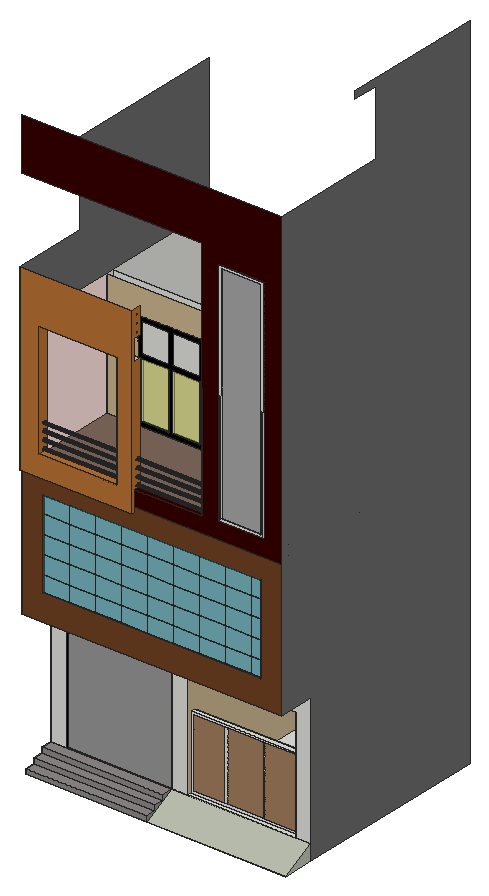
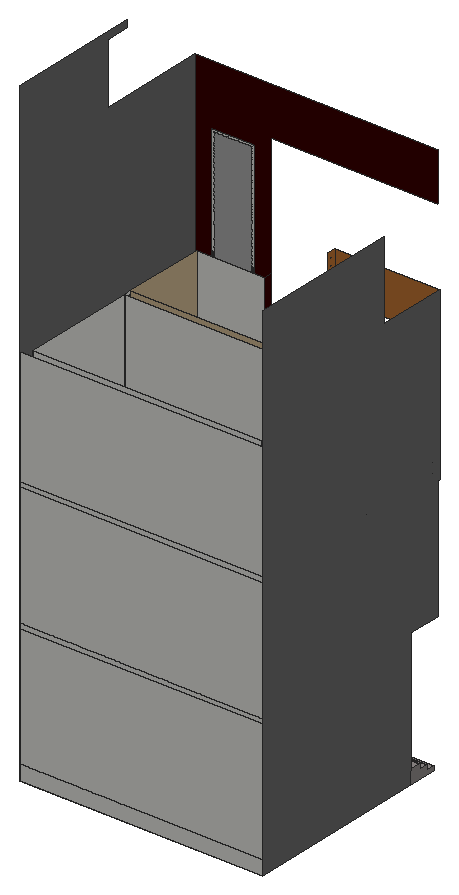
# SketchUp Ruby script. Lengths in inches.
U = 1.inch
M = Sketchup.active_model
def pt(a) = Geom::Point3d.new(a.map { |v| v * U })
def face(e, loops, mat)
  f = e.add_face(loops[0].map { |a| pt(a) })
  loops[1..].each { |l| e.add_face(l.map { |a| pt(a) }).erase! }
  f.material = f.back_material = mat if mat
  f
end
# faces: each face lists its corners as indices into pts; further lists are holes
def faces(e, pts, list, mat = nil) = list.each { |f| face(e, (f[0].is_a?(Array) ? f : [f]).map { |l| l.map { |i| pts[i] } }, mat) }
# xy, xz, yz: faces in a plane at the given z, y or x. An outline is a flat list of corners, or four numbers for a rectangle; further outlines are holes
def ring(l) = l.size == 4 ? [[l[0], l[1]], [l[2], l[1]], [l[2], l[3]], [l[0], l[3]]] : l.each_slice(2).to_a
def flat(e, list, mat, &to3) = list.each { |f| face(e, (f[0].is_a?(Array) ? f : [f]).map { |l| ring(l).map { |u, v| to3.(u, v) } }, mat) }
def xy(e, z, list, mat = nil) = flat(e, list, mat) { |x, y| [x, y, z] }
def xz(e, y, list, mat = nil) = flat(e, list, mat) { |x, z| [x, y, z] }
def yz(e, x, list, mat = nil) = flat(e, list, mat) { |y, z| [x, y, z] }
def lines(e, pts, list) = list.each { |a, b| e.add_line(pt(pts[a]), pt(pts[b])) }
# prism: a flat outline (further loops are holes) pulled along v
def prism(e, loops, v, mat = nil)
  f = face(e, loops, mat); d = Geom::Vector3d.new(v.map { |x| x * U })
  f.pushpull(f.normal.samedirection?(d) ? d.length : -d.length)
end
def box(e, o, s, mat = nil) = prism(e, [[o, [o[0] + s[0], o[1], o[2]], [o[0] + s[0], o[1] + s[1], o[2]], [o[0], o[1] + s[1], o[2]]]], [0, 0, s[2]], mat)
def at(x, y, z, deg = 0) = Geom::Transformation.translation(pt([x, y, z])) * Geom::Transformation.rotation(ORIGIN, Z_AXIS, deg.degrees)
def axes(o, x, y, z) = Geom::Transformation.new([*x, 0, *y, 0, *z, 0, *pt(o).to_a, 1])
def part(name) = M.definitions.add(name)
# library, detail: a bought-in or finely detailed component or shape, given as its bounding box
def library(name, o, s) = part(name).tap { |d| box(d.entities, o, s) }
def detail(e, o, s) = box(e.add_group.entities, o, s)
def put(e, d, t, mat = nil) = e.add_instance(d, t).tap { |i| i.material = mat if mat }
def group(e, t, mat = nil) = e.add_group.tap { |g| g.transformation = t; g.material = mat if mat }.entities
root = M.entities
M.materials.add("[0007_MistyRose]").color = [255, 228, 225]
M.materials.add("[0022_Maroon]").color = [56, 0, 0]
M.materials.add("[0032_Moccasin]").color = [204, 182, 144]
M.materials.add("[0134_DimGray]").color = [105, 105, 105]
M.materials.add("[0137_Black]").color = [0, 0, 0]
M.materials.add("[Checker Plate]").color = [168, 168, 168]
M.materials.add("[Cladding Siding Tan]").color = [162, 126, 95]
M.materials.add("[Cladding Siding White]").color = [153, 153, 153]
M.materials.add("[Granite Brown]").color = [126, 104, 91]
M.materials.add("[Metal Silver]").color = [234, 233, 238]
M.materials.add("[Pavers with Grass Brick]").color = [187, 192, 176]
M.materials.add("[Stone Marble]").color = [143, 138, 136]
M.materials.add("[Translucent Glass Gray]").color = [220, 221, 73]
M.materials["[Translucent Glass Gray]"].alpha = 0.5
M.materials.add("[Translucent Glass Tinted]").color = [5, 136, 163]
M.materials["[Translucent Glass Tinted]"].alpha = 0.48
M.materials.add("[Wood Floor Dark]").color = [186, 114, 51]
M.materials.add("[Wood Veneer 01]").color = [112, 65, 34]
xy(root,-24,[[0,17,278.8125,89],[278.8125,17,600,89],[0,89,600,545]])
xy(root,-12,[[0,17,278.8125,40.0625]],"[Stone Marble]")
xy(root,0,[[0,40.0625,278.8125,62.6875]],"[Stone Marble]")
xy(root,12,[[314.8125,89,564,99.2],[314.8125,99.2,564,109.7],[314.8125,109.7,564,533]])
xy(root,12,[[36,89,278.8125,92]],"[0137_Black]")
xy(root,12,[[0,62.6875,278.8125,89]],"[Stone Marble]")
xy(root,181.25,[[314.8125,99.2,564,109.7]])
xy(root,264,[[36,88,278.8125,92]],"[0137_Black]")
xy(root,271.23,[[314.8125,89,564,533]],"[0032_Moccasin]")
xy(root,285.55,[[36,88,278.8125,89]])
xy(root,312,[[[0,5,600,89],[163.68,35.64,166.79,36.05,169.68,37.25,172.16,39.15,174.07,41.64,175.27,44.53,175.68,47.64,175.27,50.75,174.07,53.64,172.16,56.125,169.68,58.03,166.79,59.23,163.68,59.64,160.57,59.23,157.68,58.03,155.19,56.125,153.29,53.64,152.09,50.75,151.68,47.64,152.09,44.53,153.29,41.64,155.19,39.15,157.68,37.25,160.57,36.05],[55.68,35.64,58.79,36.05,61.68,37.25,64.16,39.15,66.07,41.64,67.27,44.53,67.68,47.64,67.27,50.75,66.07,53.64,64.16,56.125,61.68,58.03,58.79,59.23,55.68,59.64,52.57,59.23,49.68,58.03,47.19,56.125,45.29,53.64,44.09,50.75,43.68,47.64,44.09,44.53,45.29,41.64,47.19,39.15,49.68,37.25,52.57,36.05],[487.68,35.64,490.79,36.05,493.68,37.25,496.16,39.15,498.07,41.64,499.27,44.53,499.68,47.64,499.27,50.75,498.07,53.64,496.16,56.125,493.68,58.03,490.79,59.23,487.68,59.64,484.57,59.23,481.68,58.03,479.19,56.125,477.29,53.64,476.09,50.75,475.68,47.64,476.09,44.53,477.29,41.64,479.19,39.15,481.68,37.25,484.57,36.05],[379.68,35.64,382.79,36.05,385.68,37.25,388.16,39.15,390.07,41.64,391.27,44.53,391.68,47.64,391.27,50.75,390.07,53.64,388.16,56.125,385.68,58.03,382.79,59.23,379.68,59.64,376.57,59.23,373.68,58.03,371.19,56.125,369.29,53.64,368.09,50.75,367.68,47.64,368.09,44.53,369.29,41.64,371.19,39.15,373.68,37.25,376.57,36.05],[271.68,35.64,274.79,36.05,277.68,37.25,280.16,39.15,282.07,41.64,283.27,44.53,283.68,47.64,283.27,50.75,282.07,53.64,280.16,56.125,277.68,58.03,274.79,59.23,271.68,59.64,268.57,59.23,265.68,58.03,263.19,56.125,261.29,53.64,260.09,50.75,259.68,47.64,260.09,44.53,261.29,41.64,263.19,39.15,265.68,37.25,268.57,36.05]],[55.68,35.64,52.57,36.05,49.68,37.25,47.19,39.15,45.29,41.64,44.09,44.53,43.68,47.64,44.09,50.75,45.29,53.64,47.19,56.125,49.68,58.03,52.57,59.23,55.68,59.64,58.79,59.23,61.68,58.03,64.16,56.125,66.07,53.64,67.27,50.75,67.68,47.64,67.27,44.53,66.07,41.64,64.16,39.15,61.68,37.25,58.79,36.05],[163.68,35.64,160.57,36.05,157.68,37.25,155.19,39.15,153.29,41.64,152.09,44.53,151.68,47.64,152.09,50.75,153.29,53.64,155.19,56.125,157.68,58.03,160.57,59.23,163.68,59.64,166.79,59.23,169.68,58.03,172.16,56.125,174.07,53.64,175.27,50.75,175.68,47.64,175.27,44.53,174.07,41.64,172.16,39.15,169.68,37.25,166.79,36.05],[271.68,35.64,268.57,36.05,265.68,37.25,263.19,39.15,261.29,41.64,260.09,44.53,259.68,47.64,260.09,50.75,261.29,53.64,263.19,56.125,265.68,58.03,268.57,59.23,271.68,59.64,274.79,59.23,277.68,58.03,280.16,56.125,282.07,53.64,283.27,50.75,283.68,47.64,283.27,44.53,282.07,41.64,280.16,39.15,277.68,37.25,274.79,36.05],[379.68,35.64,376.57,36.05,373.68,37.25,371.19,39.15,369.29,41.64,368.09,44.53,367.68,47.64,368.09,50.75,369.29,53.64,371.19,56.125,373.68,58.03,376.57,59.23,379.68,59.64,382.79,59.23,385.68,58.03,388.16,56.125,390.07,53.64,391.27,50.75,391.68,47.64,391.27,44.53,390.07,41.64,388.16,39.15,385.68,37.25,382.79,36.05],
  [487.68,35.64,484.57,36.05,481.68,37.25,479.19,39.15,477.29,41.64,476.09,44.53,475.68,47.64,476.09,50.75,477.29,53.64,479.19,56.125,481.68,58.03,484.57,59.23,487.68,59.64,490.79,59.23,493.68,58.03,496.16,56.125,498.07,53.64,499.27,50.75,499.68,47.64,499.27,44.53,498.07,41.64,496.16,39.15,493.68,37.25,490.79,36.05]])
xy(root,324,[[18,23,582,527]])
xy(root,372,[[48,5,552,8]],"[Wood Veneer 01]")
xy(root,576,[[48,5,552,8]],"[Wood Veneer 01]")
xy(root,612,[[0,0,258,5]],"[Wood Floor Dark]")
xy(root,636,[[18,227,582,245],[18,245,582,527]])
xy(root,636,[[18,23,582,227]],"[Granite Brown]")
xy(root,645.8125,[[98.58,227,160.58,229],[170.58,227,232.58,229],[242.58,227,307.71,229]])
xy(root,660,[[258,5,414,23]],"[0022_Maroon]")
xy(root,660,[[42,0,222,23]],"[Wood Floor Dark]")
xy(root,665.86,[[455.86,3,558.14,5]])
xy(root,670.74,[[460.74,3,553.26,5]])
xy(root,704.4,[[370.68,227,426.27,229],[434.59,227,482.8,229]])
xz(root,0,[[[0,612,258,1032],[42,660,222,924]]],"[Wood Floor Dark]")
xz(root,3,[[[455.86,665.86,558.14,1194.14],[460.74,670.74,553.26,1189.26]]])
xz(root,5,[[[455.86,665.86,558.14,1194.14],[460.74,670.74,553.26,1189.26]]])
xz(root,5,[[[258,624,600,624,600,1344,0,1344,0,1224,414,1224,414,660,258,660],[455.86,665.86,558.14,1194.14]]],"[0022_Maroon]")
xz(root,5,[[460.74,670.74,553.26,1189.26]],"[Checker Plate]")
xz(root,5,[[[0,312,600,312,600,624,258,624,258,612,0,612],[48,372,552,576]]],"[Wood Veneer 01]")
xz(root,8,[[48,372,108,408],[108,372,168,408],[168,372,228,408],[228,372,288,408],[288,372,348,408],
  [348,372,408,408],[408,372,468,408],[468,372,528,408],[528,372,552,408],[48,408,108,450],
  [108,408,168,450],[168,408,228,450],[228,408,288,450],[288,408,348,450],[348,408,408,450],
  [408,408,468,450],[468,408,528,450],[528,408,552,450],[48,450,108,492],[108,450,168,492],
  [168,450,228,492],[228,450,288,492],[288,450,348,492],[348,450,408,492],[408,450,468,492],
  [468,450,528,492],[528,450,552,492],[48,492,108,534],[108,492,168,534],[168,492,228,534],
  [228,492,288,534],[288,492,348,534],[348,492,408,534],[408,492,468,534],[468,492,528,534],
  [528,492,552,534],[48,534,108,576],[108,534,168,576],[168,534,228,576],[228,534,288,576],
  [288,534,348,576],[348,534,408,576],[408,534,468,576],[468,534,528,576],[528,534,552,576]],"[Translucent Glass Tinted]")
xz(root,17,[[0,-24,278.8125,-12]],"[Stone Marble]")
xz(root,23,[[18,324,582,624],[18,636,582,660],[18,660,42,924],[222,660,258,924],[414,660,582,924]])
xz(root,40.0625,[[0,-12,278.8125,0]],"[Stone Marble]")
xz(root,62.6875,[[0,0,278.8125,12]],"[Stone Marble]")
xz(root,88,[[36,264,278.8125,285.55]],"[0137_Black]")
xz(root,89,[[0,-24,278.8125,-12],[278.8125,-24,600,12],[0,-12,278.8125,0],[0,0,278.8125,12],[0,12,36,12,36,285.55,278.8125,285.55,278.8125,12,314.8125,12,314.8125,271.23,564,271.23,564,12,600,12,600,312,0,312]])
xz(root,92,[[36,12,278.8125,264]],"[Cladding Siding White]")
xz(root,99.2,[[392.8125,18,398.8125,175.25]])
xz(root,99.2,[[320.8125,18,392.8125,175.25],[398.8125,18,479.75,175.25],[485.75,18,558,175.25]],"[Cladding Siding Tan]")
xz(root,99.2,[[[314.8125,12,564,181.25],[320.8125,18,558,175.25]],[479.75,18,485.75,175.25]],"[Metal Silver]")
xz(root,109.7,[[314.8125,12,564,181.25]])
xz(root,227,[[[18,636,88.77,636,88.77,864.75,317.52,864.75,317.52,636,582,636,582,924,18,924],[361.58,695.31,491.89,865.62]]],"[0032_Moccasin]")
xz(root,227,[[[88.77,636,317.52,864.75],[242.58,645.8125,307.71,776.75],[98.58,645.8125,160.58,776.75],[170.58,645.8125,232.58,776.75],[242.58,786.75,307.71,854.9375],[170.58,786.75,232.58,854.9375],[98.58,786.75,160.58,854.9375]],[[361.58,695.31,491.89,865.62],[370.68,704.4,482.8,856.52]],[426.27,704.4,434.59,856.52]],"[0137_Black]")
xz(root,229,[[98.58,645.8125,160.58,776.75],[170.58,645.8125,232.58,776.75],[242.58,645.8125,307.71,776.75],[370.68,704.4,426.27,856.52],[434.59,704.4,482.8,856.52]],"[Translucent Glass Gray]")
xz(root,245,[[18,636,582,924]])
xz(root,527,[[18,324,582,624],[18,636,582,924]])
xz(root,533,[[314.8125,12,564,271.23]],"[0032_Moccasin]")
xz(root,545,[[0,-24,600,12],[0,12,600,312],[0,312,600,324],[0,324,600,624],[0,624,600,636],
  [0,636,600,924]])
yz(root,0,[[89,-24,89,312,5,312,5,612,0,612,0,1032,173,1032,173,1224,545,1224,545,-24]],"[0134_DimGray]")
yz(root,0,[[17,-24,17,-12,40.0625,-12,40.0625,0,62.6875,0,62.6875,12,89,12,89,-24]],"[Stone Marble]")
yz(root,18,[[23,324,527,624],[227,636,245,924],[245,636,527,924]])
yz(root,18,[[23,636,227,924]],"[0007_MistyRose]")
yz(root,36,[[88,264,89,285.55]])
yz(root,36,[[89,12,92,264]],"[0137_Black]")
yz(root,42,[[14,663,13.22,663.1,12.5,663.4,11.88,663.88,11.4,664.5,11.1,665.22,11,666,11.1,666.78,11.4,667.5,11.88,668.12,12.5,668.6,13.22,668.9,14,669,14.78,668.9,15.5,668.6,16.12,668.12,16.6,667.5,16.9,666.78,17,666,16.9,665.22,16.6,664.5,16.12,663.88,15.5,663.4,14.78,663.1],[14,681,13.22,681.1,12.5,681.4,11.88,681.88,11.4,682.5,11.1,683.22,11,684,11.1,684.78,11.4,685.5,11.88,686.12,12.5,686.6,13.22,686.9,14,687,14.78,686.9,15.5,686.6,16.12,686.12,16.6,685.5,16.9,684.78,17,684,16.9,683.22,16.6,682.5,16.12,681.88,15.5,681.4,14.78,681.1],[14,699,13.22,699.1,12.5,699.4,11.88,699.88,11.4,700.5,11.1,701.22,11,702,11.1,702.78,11.4,703.5,11.88,704.12,12.5,704.6,13.22,704.9,14,705,14.78,704.9,15.5,704.6,16.12,704.12,16.6,703.5,16.9,702.78,17,702,16.9,701.22,16.6,700.5,16.12,699.88,15.5,699.4,14.78,699.1],[14,717,13.22,717.1,12.5,717.4,11.88,717.88,11.4,718.5,11.1,719.22,11,720,11.1,720.78,11.4,721.5,11.88,722.12,12.5,722.6,13.22,722.9,14,723,14.78,722.9,15.5,722.6,16.12,722.12,16.6,721.5,16.9,720.78,17,720,16.9,719.22,16.6,718.5,16.12,717.88,15.5,717.4,14.78,717.1]])
yz(root,42,[[[0,660,23,924],[14,717,13.22,717.1,12.5,717.4,11.88,717.88,11.4,718.5,11.1,719.22,11,720,11.1,720.78,11.4,721.5,11.88,722.12,12.5,722.6,13.22,722.9,14,723,14.78,722.9,15.5,722.6,16.12,722.12,16.6,721.5,16.9,720.78,17,720,16.9,719.22,16.6,718.5,16.12,717.88,15.5,717.4,14.78,717.1],[14,699,13.22,699.1,12.5,699.4,11.88,699.88,11.4,700.5,11.1,701.22,11,702,11.1,702.78,11.4,703.5,11.88,704.12,12.5,704.6,13.22,704.9,14,705,14.78,704.9,15.5,704.6,16.12,704.12,16.6,703.5,16.9,702.78,17,702,16.9,701.22,16.6,700.5,16.12,699.88,15.5,699.4,14.78,699.1],[14,681,13.22,681.1,12.5,681.4,11.88,681.88,11.4,682.5,11.1,683.22,11,684,11.1,684.78,11.4,685.5,11.88,686.12,12.5,686.6,13.22,686.9,14,687,14.78,686.9,15.5,686.6,16.12,686.12,16.6,685.5,16.9,684.78,17,684,16.9,683.22,16.6,682.5,16.12,681.88,15.5,681.4,14.78,681.1],[14,663,13.22,663.1,12.5,663.4,11.88,663.88,11.4,664.5,11.1,665.22,11,666,11.1,666.78,11.4,667.5,11.88,668.12,12.5,668.6,13.22,668.9,14,669,14.78,668.9,15.5,668.6,16.12,668.12,16.6,667.5,16.9,666.78,17,666,16.9,665.22,16.6,664.5,16.12,663.88,15.5,663.4,14.78,663.1]]],"[Wood Floor Dark]")
yz(root,48,[[5,372,8,576]],"[Wood Veneer 01]")
yz(root,98.58,[[227,645.8125,229,776.75]])
yz(root,160.58,[[227,645.8125,229,776.75]])
yz(root,170.58,[[227,645.8125,229,776.75]])
yz(root,222,[[[0,660,23,924],[14,717,14.78,717.1,15.5,717.4,16.12,717.88,16.6,718.5,16.9,719.22,17,720,16.9,720.78,16.6,721.5,16.12,722.12,15.5,722.6,14.78,722.9,14,723,13.22,722.9,12.5,722.6,11.88,722.12,11.4,721.5,11.1,720.78,11,720,11.1,719.22,11.4,718.5,11.88,717.88,12.5,717.4,13.22,717.1],[14,699,14.78,699.1,15.5,699.4,16.12,699.88,16.6,700.5,16.9,701.22,17,702,16.9,702.78,16.6,703.5,16.12,704.12,15.5,704.6,14.78,704.9,14,705,13.22,704.9,12.5,704.6,11.88,704.12,11.4,703.5,11.1,702.78,11,702,11.1,701.22,11.4,700.5,11.88,699.88,12.5,699.4,13.22,699.1],[14,681,14.78,681.1,15.5,681.4,16.12,681.88,16.6,682.5,16.9,683.22,17,684,16.9,684.78,16.6,685.5,16.12,686.12,15.5,686.6,14.78,686.9,14,687,13.22,686.9,12.5,686.6,11.88,686.12,11.4,685.5,11.1,684.78,11,684,11.1,683.22,11.4,682.5,11.88,681.88,12.5,681.4,13.22,681.1],[14,663,14.78,663.1,15.5,663.4,16.12,663.88,16.6,664.5,16.9,665.22,17,666,16.9,666.78,16.6,667.5,16.12,668.12,15.5,668.6,14.78,668.9,14,669,13.22,668.9,12.5,668.6,11.88,668.12,11.4,667.5,11.1,666.78,11,666,11.1,665.22,11.4,664.5,11.88,663.88,12.5,663.4,13.22,663.1]]],"[Wood Floor Dark]")
yz(root,232.58,[[227,645.8125,229,776.75]])
yz(root,242.58,[[227,645.8125,229,776.75]])
yz(root,258,[[14,663,13.22,663.1,12.5,663.4,11.88,663.88,11.4,664.5,11.1,665.22,11,666,11.1,666.78,11.4,667.5,11.88,668.12,12.5,668.6,13.22,668.9,14,669,14.78,668.9,15.5,668.6,16.12,668.12,16.6,667.5,16.9,666.78,17,666,16.9,665.22,16.6,664.5,16.12,663.88,15.5,663.4,14.78,663.1],[14,681,13.22,681.1,12.5,681.4,11.88,681.88,11.4,682.5,11.1,683.22,11,684,11.1,684.78,11.4,685.5,11.88,686.12,12.5,686.6,13.22,686.9,14,687,14.78,686.9,15.5,686.6,16.12,686.12,16.6,685.5,16.9,684.78,17,684,16.9,683.22,16.6,682.5,16.12,681.88,15.5,681.4,14.78,681.1],[14,699,13.22,699.1,12.5,699.4,11.88,699.88,11.4,700.5,11.1,701.22,11,702,11.1,702.78,11.4,703.5,11.88,704.12,12.5,704.6,13.22,704.9,14,705,14.78,704.9,15.5,704.6,16.12,704.12,16.6,703.5,16.9,702.78,17,702,16.9,701.22,16.6,700.5,16.12,699.88,15.5,699.4,14.78,699.1],[14,717,13.22,717.1,12.5,717.4,11.88,717.88,11.4,718.5,11.1,719.22,11,720,11.1,720.78,11.4,721.5,11.88,722.12,12.5,722.6,13.22,722.9,14,723,14.78,722.9,15.5,722.6,16.12,722.12,16.6,721.5,16.9,720.78,17,720,16.9,719.22,16.6,718.5,16.12,717.88,15.5,717.4,14.78,717.1]])
yz(root,258,[[[0,612,5,612,5,660,23,660,23,924,5,924,5,972,23,972,23,1032,0,1032],[14,977.83,13.63,977.85,13.27,977.91,12.92,978,12.57,978.14,12.25,978.3,11.9375,978.5,11.65,978.73,11.39,978.99,11.16,979.28,10.96,979.59,10.8,979.91,10.66,980.26,10.57,980.61,10.51,980.97,10.49,981.34,10.51,981.71,10.57,982.07,10.66,982.42,10.8,982.77,10.96,983.09,11.16,983.4,11.39,983.6875,11.65,983.95,11.9375,984.18,12.25,984.38,12.57,984.54,12.92,984.68,13.27,984.77,13.63,984.83,14,984.85,14.37,984.83,14.73,984.77,15.08,984.68,15.43,984.54,15.75,984.38,16.0625,984.18,16.35,983.95,16.61,983.6875,16.84,983.4,17.04,983.09,17.2,982.77,17.34,982.42,17.43,982.07,17.49,981.71,17.51,981.34,17.49,980.97,17.43,980.61,17.34,980.26,17.2,979.91,17.04,979.59,16.84,979.28,16.61,978.99,16.35,978.73,16.0625,978.5,15.75,978.3,15.43,978.14,15.08,978,14.73,977.91,14.37,977.85],[14,1013.83,13.63,1013.85,13.27,1013.91,12.92,1014.01,12.57,1014.14,12.25,1014.3,11.9375,1014.5,11.65,1014.74,11.39,1014.99,11.16,1015.28,10.96,1015.59,10.8,1015.91,10.67,1016.26,10.57,1016.61,10.51,1016.97,10.49,1017.34,10.51,1017.71,10.57,1018.07,10.67,1018.42,10.8,1018.77,10.96,1019.09,11.16,1019.4,11.39,1019.6875,11.65,1019.95,11.9375,1020.18,12.25,1020.375,12.57,1020.54,12.92,1020.68,13.27,1020.77,13.63,1020.83,14,1020.85,14.37,1020.83,14.73,1020.77,15.08,1020.68,15.43,1020.54,15.75,1020.375,16.0625,1020.18,16.35,1019.95,16.61,1019.6875,16.84,1019.4,17.04,1019.09,17.2,1018.77,17.33,1018.42,17.43,1018.07,17.49,1017.71,17.51,1017.34,17.49,1016.97,17.43,1016.61,17.33,1016.26,17.2,1015.91,17.04,1015.59,16.84,1015.28,16.61,1014.99,16.35,1014.74,16.0625,1014.5,15.75,1014.3,15.43,1014.14,15.08,1014.01,14.73,1013.91,14.37,1013.85],[14,996.07,13.66,996.09,13.32,996.14,12.99,996.23,12.67,996.35,12.36,996.51,12.08,996.69,11.81,996.91,11.57,997.15,11.35,997.42,11.17,997.7,11.01,998.01,10.89,998.33,10.8,998.66,10.75,999,10.73,999.34,10.75,999.68,10.8,1000.02,10.89,1000.35,11.01,1000.67,11.17,1000.98,11.35,1001.26,11.57,1001.53,11.81,1001.77,12.08,1001.99,12.36,1002.17,12.67,1002.33,12.99,1002.45,13.32,1002.54,13.66,1002.6,14,1002.61,14.34,1002.6,14.68,1002.54,15.01,1002.45,15.33,1002.33,15.64,1002.17,15.92,1001.99,16.19,1001.77,16.43,1001.53,16.65,1001.26,16.83,1000.98,16.99,1000.67,17.11,1000.35,17.2,1000.02,17.25,999.68,17.27,999.34,17.25,999,17.2,998.66,17.11,998.33,16.99,998.01,16.83,997.7,16.65,997.42,16.43,997.15,16.19,996.91,15.92,996.69,15.64,996.51,15.33,996.35,15.01,996.23,14.68,996.14,14.34,996.09],[14,717,13.22,717.1,12.5,717.4,11.88,717.88,11.4,718.5,11.1,719.22,11,720,11.1,720.78,11.4,721.5,11.88,722.12,12.5,722.6,13.22,722.9,14,723,14.78,722.9,15.5,722.6,16.12,722.12,16.6,721.5,16.9,720.78,17,720,16.9,719.22,16.6,718.5,16.12,717.88,15.5,717.4,14.78,717.1],[14,699,13.22,699.1,12.5,699.4,11.88,699.88,11.4,700.5,11.1,701.22,11,702,11.1,702.78,11.4,703.5,11.88,704.12,12.5,704.6,13.22,704.9,14,705,14.78,704.9,15.5,704.6,16.12,704.12,16.6,703.5,16.9,702.78,17,702,16.9,701.22,16.6,700.5,16.12,699.88,15.5,699.4,14.78,699.1],[14,681,13.22,681.1,12.5,681.4,11.88,681.88,11.4,682.5,11.1,683.22,11,684,11.1,684.78,11.4,685.5,11.88,686.12,12.5,686.6,13.22,686.9,14,687,14.78,686.9,15.5,686.6,16.12,686.12,16.6,685.5,16.9,684.78,17,684,16.9,683.22,16.6,682.5,16.12,681.88,15.5,681.4,14.78,681.1],[14,663,13.22,663.1,12.5,663.4,11.88,663.88,11.4,664.5,11.1,665.22,11,666,11.1,666.78,11.4,667.5,11.88,668.12,12.5,668.6,13.22,668.9,14,669,14.78,668.9,15.5,668.6,16.12,668.12,16.6,667.5,16.9,666.78,17,666,16.9,665.22,16.6,664.5,16.12,663.88,15.5,663.4,14.78,663.1]]],"[Wood Floor Dark]")
yz(root,278.8125,[[88,264,89,285.55]])
yz(root,278.8125,[[89,12,92,264]],"[0137_Black]")
yz(root,278.8125,[[17,-24,89,12,62.6875,12,62.6875,0,40.0625,0,40.0625,-12,17,-12]],"[Stone Marble]")
yz(root,307.71,[[227,645.8125,229,776.75]])
yz(root,314.8125,[[89,12,99.2,12,99.2,181.25,109.7,181.25,109.7,12,533,12,533,271.23,89,271.23]],"[0032_Moccasin]")
yz(root,370.68,[[227,704.4,229,856.52]])
yz(root,414,[[[5,660,23,924],[14,717,14.78,717.1,15.5,717.4,16.12,717.88,16.6,718.5,16.9,719.22,17,720,16.9,720.78,16.6,721.5,16.12,722.12,15.5,722.6,14.78,722.9,14,723,13.22,722.9,12.5,722.6,11.88,722.12,11.4,721.5,11.1,720.78,11,720,11.1,719.22,11.4,718.5,11.88,717.88,12.5,717.4,13.22,717.1],[14,699,14.78,699.1,15.5,699.4,16.12,699.88,16.6,700.5,16.9,701.22,17,702,16.9,702.78,16.6,703.5,16.12,704.12,15.5,704.6,14.78,704.9,14,705,13.22,704.9,12.5,704.6,11.88,704.12,11.4,703.5,11.1,702.78,11,702,11.1,701.22,11.4,700.5,11.88,699.88,12.5,699.4,13.22,699.1],[14,681,14.78,681.1,15.5,681.4,16.12,681.88,16.6,682.5,16.9,683.22,17,684,16.9,684.78,16.6,685.5,16.12,686.12,15.5,686.6,14.78,686.9,14,687,13.22,686.9,12.5,686.6,11.88,686.12,11.4,685.5,11.1,684.78,11,684,11.1,683.22,11.4,682.5,11.88,681.88,12.5,681.4,13.22,681.1],[14,663,14.78,663.1,15.5,663.4,16.12,663.88,16.6,664.5,16.9,665.22,17,666,16.9,666.78,16.6,667.5,16.12,668.12,15.5,668.6,14.78,668.9,14,669,13.22,668.9,12.5,668.6,11.88,668.12,11.4,667.5,11.1,666.78,11,666,11.1,665.22,11.4,664.5,11.88,663.88,12.5,663.4,13.22,663.1]]],"[0022_Maroon]")
yz(root,426.27,[[227,704.4,229,856.52]])
yz(root,434.59,[[227,704.4,229,856.52]])
yz(root,455.86,[[3,665.86,5,924]])
yz(root,460.74,[[3,670.74,5,924]])
yz(root,482.8,[[227,704.4,229,856.52]])
yz(root,552,[[5,372,8,576]],"[Wood Veneer 01]")
yz(root,553.26,[[3,670.74,5,924]])
yz(root,558.14,[[3,665.86,5,924]])
yz(root,564,[[99.2,12,109.7,181.25]])
yz(root,564,[[89,12,89,271.23,533,271.23,533,12,109.7,12,109.7,181.25,99.2,181.25,99.2,12]],"[0032_Moccasin]")
yz(root,582,[[23,324,527,624],[227,636,245,924],[245,636,527,924]])
yz(root,582,[[23,636,227,924]],"[0032_Moccasin]")
yz(root,600,[[89,-24,545,-24,545,1512,215,1512,215,1494,275,1494,275,1344,5,1344,5,312,89,312]],"[0134_DimGray]")
yz(root,600,[[17,-24,89,-24,89,12]],"[Pavers with Grass Brick]")
p = [[600,17,-24],[600,89,12],[564,89,12],[314.8125,89,12],[278.8125,89,12],[278.8125,17,-24],
  [42,13.22,663.1],[42,14,663],[222,14,663],[222,13.22,663.1],[258,13.22,663.1],[258,14,663],
  [414,14,663],[414,13.22,663.1],[42,14.78,663.1],[222,14.78,663.1],[258,14.78,663.1],[414,14.78,663.1],
  [42,12.5,663.4],[222,12.5,663.4],[258,12.5,663.4],[414,12.5,663.4],[42,15.5,663.4],[222,15.5,663.4],
  [258,15.5,663.4],[414,15.5,663.4],[42,11.88,663.88],[222,11.88,663.88],[258,11.88,663.88],[414,11.88,663.88],
  [42,16.12,663.88],[222,16.12,663.88],[258,16.12,663.88],[414,16.12,663.88],[42,11.4,664.5],[222,11.4,664.5],
  [258,11.4,664.5],[414,11.4,664.5],[42,16.6,664.5],[222,16.6,664.5],[258,16.6,664.5],[414,16.6,664.5],
  [42,11.1,665.22],[222,11.1,665.22],[258,11.1,665.22],[414,11.1,665.22],[42,16.9,665.22],[222,16.9,665.22],
  [258,16.9,665.22],[414,16.9,665.22],[42,11,666],[222,11,666],[258,11,666],[414,11,666],
  [42,17,666],[222,17,666],[258,17,666],[414,17,666],[42,11.1,666.78],[222,11.1,666.78],
  [258,11.1,666.78],[414,11.1,666.78],[42,16.9,666.78],[222,16.9,666.78],[258,16.9,666.78],[414,16.9,666.78],
  [42,11.4,667.5],[222,11.4,667.5],[258,11.4,667.5],[414,11.4,667.5],[42,16.6,667.5],[222,16.6,667.5],
  [258,16.6,667.5],[414,16.6,667.5],[42,11.88,668.12],[222,11.88,668.12],[258,11.88,668.12],[414,11.88,668.12],
  [42,16.12,668.12],[222,16.12,668.12],[258,16.12,668.12],[414,16.12,668.12],[42,12.5,668.6],[222,12.5,668.6],
  [258,12.5,668.6],[414,12.5,668.6],[42,15.5,668.6],[222,15.5,668.6],[258,15.5,668.6],[414,15.5,668.6],
  [42,13.22,668.9],[222,13.22,668.9],[258,13.22,668.9],[414,13.22,668.9],[42,14.78,668.9],[222,14.78,668.9],
  [258,14.78,668.9],[414,14.78,668.9],[42,14,669],[222,14,669],[258,14,669],[414,14,669],
  [42,13.22,681.1],[42,14,681],[222,14,681],[222,13.22,681.1],[258,13.22,681.1],[258,14,681],
  [414,14,681],[414,13.22,681.1],[42,14.78,681.1],[222,14.78,681.1],[258,14.78,681.1],[414,14.78,681.1],
  [42,12.5,681.4],[222,12.5,681.4],[258,12.5,681.4],[414,12.5,681.4],[42,15.5,681.4],[222,15.5,681.4],
  [258,15.5,681.4],[414,15.5,681.4],[42,11.88,681.88],[222,11.88,681.88],[258,11.88,681.88],[414,11.88,681.88],
  [42,16.12,681.88],[222,16.12,681.88],[258,16.12,681.88],[414,16.12,681.88],[42,11.4,682.5],[222,11.4,682.5],
  [258,11.4,682.5],[414,11.4,682.5],[42,16.6,682.5],[222,16.6,682.5],[258,16.6,682.5],[414,16.6,682.5],
  [42,11.1,683.22],[222,11.1,683.22],[258,11.1,683.22],[414,11.1,683.22],[42,16.9,683.22],[222,16.9,683.22],
  [258,16.9,683.22],[414,16.9,683.22],[42,11,684],[222,11,684],[258,11,684],[414,11,684],
  [42,17,684],[222,17,684],[258,17,684],[414,17,684],[42,11.1,684.78],[222,11.1,684.78],
  [258,11.1,684.78],[414,11.1,684.78],[42,16.9,684.78],[222,16.9,684.78],[258,16.9,684.78],[414,16.9,684.78],
  [42,11.4,685.5],[222,11.4,685.5],[258,11.4,685.5],[414,11.4,685.5],[42,16.6,685.5],[222,16.6,685.5],
  [258,16.6,685.5],[414,16.6,685.5],[42,11.88,686.12],[222,11.88,686.12],[258,11.88,686.12],[414,11.88,686.12],
  [42,16.12,686.12],[222,16.12,686.12],[258,16.12,686.12],[414,16.12,686.12],[42,12.5,686.6],[222,12.5,686.6],
  [258,12.5,686.6],[414,12.5,686.6],[42,15.5,686.6],[222,15.5,686.6],[258,15.5,686.6],[414,15.5,686.6],
  [42,13.22,686.9],[222,13.22,686.9],[258,13.22,686.9],[414,13.22,686.9],[42,14.78,686.9],[222,14.78,686.9],
  [258,14.78,686.9],[414,14.78,686.9],[42,14,687],[222,14,687],[258,14,687],[414,14,687],
  [42,13.22,699.1],[42,14,699],[222,14,699],[222,13.22,699.1],[258,13.22,699.1],[258,14,699],
  [414,14,699],[414,13.22,699.1],[42,14.78,699.1],[222,14.78,699.1],[258,14.78,699.1],[414,14.78,699.1],
  [42,12.5,699.4],[222,12.5,699.4],[258,12.5,699.4],[414,12.5,699.4],[42,15.5,699.4],[222,15.5,699.4],
  [258,15.5,699.4],[414,15.5,699.4],[42,11.88,699.88],[222,11.88,699.88],[258,11.88,699.88],[414,11.88,699.88],
  [42,16.12,699.88],[222,16.12,699.88],[258,16.12,699.88],[414,16.12,699.88],[42,11.4,700.5],[222,11.4,700.5],
  [258,11.4,700.5],[414,11.4,700.5],[42,16.6,700.5],[222,16.6,700.5],[258,16.6,700.5],[414,16.6,700.5],
  [42,11.1,701.22],[222,11.1,701.22],[258,11.1,701.22],[414,11.1,701.22],[42,16.9,701.22],[222,16.9,701.22],
  [258,16.9,701.22],[414,16.9,701.22],[42,11,702],[222,11,702],[258,11,702],[414,11,702],
  [42,17,702],[222,17,702],[258,17,702],[414,17,702],[42,11.1,702.78],[222,11.1,702.78],
  [258,11.1,702.78],[414,11.1,702.78],[42,16.9,702.78],[222,16.9,702.78],[258,16.9,702.78],[414,16.9,702.78],
  [42,11.4,703.5],[222,11.4,703.5],[258,11.4,703.5],[414,11.4,703.5],[42,16.6,703.5],[222,16.6,703.5],
  [258,16.6,703.5],[414,16.6,703.5],[42,11.88,704.12],[222,11.88,704.12],[258,11.88,704.12],[414,11.88,704.12],
  [42,16.12,704.12],[222,16.12,704.12],[258,16.12,704.12],[414,16.12,704.12],[42,12.5,704.6],[222,12.5,704.6],
  [258,12.5,704.6],[414,12.5,704.6],[42,15.5,704.6],[222,15.5,704.6],[258,15.5,704.6],[414,15.5,704.6],
  [42,13.22,704.9],[222,13.22,704.9],[258,13.22,704.9],[414,13.22,704.9],[42,14.78,704.9],[222,14.78,704.9],
  [258,14.78,704.9],[414,14.78,704.9],[42,14,705],[222,14,705],[258,14,705],[414,14,705],
  [42,13.22,717.1],[42,14,717],[222,14,717],[222,13.22,717.1],[258,13.22,717.1],[258,14,717],
  [414,14,717],[414,13.22,717.1],[42,14.78,717.1],[222,14.78,717.1],[258,14.78,717.1],[414,14.78,717.1],
  [42,12.5,717.4],[222,12.5,717.4],[258,12.5,717.4],[414,12.5,717.4],[42,15.5,717.4],[222,15.5,717.4],
  [258,15.5,717.4],[414,15.5,717.4],[42,11.88,717.88],[222,11.88,717.88],[258,11.88,717.88],[414,11.88,717.88],
  [42,16.12,717.88],[222,16.12,717.88],[258,16.12,717.88],[414,16.12,717.88],[42,11.4,718.5],[222,11.4,718.5],
  [258,11.4,718.5],[414,11.4,718.5],[42,16.6,718.5],[222,16.6,718.5],[258,16.6,718.5],[414,16.6,718.5],
  [42,11.1,719.22],[222,11.1,719.22],[258,11.1,719.22],[414,11.1,719.22],[42,16.9,719.22],[222,16.9,719.22],
  [258,16.9,719.22],[414,16.9,719.22],[42,11,720],[222,11,720],[258,11,720],[414,11,720],
  [42,17,720],[222,17,720],[258,17,720],[414,17,720],[42,11.1,720.78],[222,11.1,720.78],
  [258,11.1,720.78],[414,11.1,720.78],[42,16.9,720.78],[222,16.9,720.78],[258,16.9,720.78],[414,16.9,720.78],
  [42,11.4,721.5],[222,11.4,721.5],[258,11.4,721.5],[414,11.4,721.5],[42,16.6,721.5],[222,16.6,721.5],
  [258,16.6,721.5],[414,16.6,721.5],[42,11.88,722.12],[222,11.88,722.12],[258,11.88,722.12],[414,11.88,722.12],
  [42,16.12,722.12],[222,16.12,722.12],[258,16.12,722.12],[414,16.12,722.12],[18,23,636],[0,23,636],
  [582,23,636],[600,23,636],[0,227,636],[18,227,636],[582,227,636],[600,227,636],
  [582,23,660],[600,23,660],[18,23,660],[0,23,660],[588,8,372],[588,8,576],
  [258,14,666],[414,14,666],[258,14,684],[414,14,684],[258,14,702],[414,14,702],
  [258,14,720],[414,14,720],[42,14,666],[222,14,666],[42,14,684],[222,14,684],
  [42,14,702],[222,14,702],[42,14,720],[222,14,720]]
faces(root,p,[[0,1,2,3,4,5]],"[Pavers with Grass Brick]")
faces(root,p,[[6,7,8,9],[10,11,12,13],[7,14,15,8],[11,16,17,12],[18,6,9,19],[20,10,13,21],[14,22,23,15],[16,24,25,17],
  [26,18,19,27],[28,20,21,29],[22,30,31,23],[24,32,33,25],[34,26,27,35],[36,28,29,37],[30,38,39,31],[32,40,41,33],
  [42,34,35,43],[44,36,37,45],[38,46,47,39],[40,48,49,41],[50,42,43,51],[52,44,45,53],[46,54,55,47],[48,56,57,49],
  [58,50,51,59],[60,52,53,61],[54,62,63,55],[56,64,65,57],[66,58,59,67],[68,60,61,69],[62,70,71,63],[64,72,73,65],
  [74,66,67,75],[76,68,69,77],[70,78,79,71],[72,80,81,73],[82,74,75,83],[84,76,77,85],[78,86,87,79],[80,88,89,81],
  [90,82,83,91],[92,84,85,93],[86,94,95,87],[88,96,97,89],[98,90,91,99],[100,92,93,101],[94,98,99,95],[96,100,101,97],
  [102,103,104,105],[106,107,108,109],[103,110,111,104],[107,112,113,108],[114,102,105,115],[116,106,109,117],[110,118,119,111],[112,120,121,113],
  [122,114,115,123],[124,116,117,125],[118,126,127,119],[120,128,129,121],[130,122,123,131],[132,124,125,133],[126,134,135,127],[128,136,137,129],
  [138,130,131,139],[140,132,133,141],[134,142,143,135],[136,144,145,137],[146,138,139,147],[148,140,141,149],[142,150,151,143],[144,152,153,145],
  [154,146,147,155],[156,148,149,157],[150,158,159,151],[152,160,161,153],[162,154,155,163],[164,156,157,165],[158,166,167,159],[160,168,169,161],
  [170,162,163,171],[172,164,165,173],[166,174,175,167],[168,176,177,169],[178,170,171,179],[180,172,173,181],[174,182,183,175],[176,184,185,177],
  [186,178,179,187],[188,180,181,189],[182,190,191,183],[184,192,193,185],[194,186,187,195],[196,188,189,197],[190,194,195,191],[192,196,197,193],
  [198,199,200,201],[202,203,204,205],[199,206,207,200],[203,208,209,204],[210,198,201,211],[212,202,205,213],[206,214,215,207],[208,216,217,209],
  [218,210,211,219],[220,212,213,221],[214,222,223,215],[216,224,225,217],[226,218,219,227],[228,220,221,229],[222,230,231,223],[224,232,233,225],
  [234,226,227,235],[236,228,229,237],[230,238,239,231],[232,240,241,233],[242,234,235,243],[244,236,237,245],[238,246,247,239],[240,248,249,241],
  [250,242,243,251],[252,244,245,253],[246,254,255,247],[248,256,257,249],[258,250,251,259],[260,252,253,261],[254,262,263,255],[256,264,265,257],
  [266,258,259,267],[268,260,261,269],[262,270,271,263],[264,272,273,265],[274,266,267,275],[276,268,269,277],[270,278,279,271],[272,280,281,273],
  [282,274,275,283],[284,276,277,285],[278,286,287,279],[280,288,289,281],[290,282,283,291],[292,284,285,293],[286,290,291,287],[288,292,293,289],
  [294,295,296,297],[298,299,300,301],[295,302,303,296],[299,304,305,300],[306,294,297,307],[308,298,301,309],[302,310,311,303],[304,312,313,305],
  [314,306,307,315],[316,308,309,317],[310,318,319,311],[312,320,321,313],[322,314,315,323],[324,316,317,325],[318,326,327,319],[320,328,329,321],
  [330,322,323,331],[332,324,325,333],[326,334,335,327],[328,336,337,329],[338,330,331,339],[340,332,333,341],[334,342,343,335],[336,344,345,337],
  [346,338,339,347],[348,340,341,349],[342,350,351,343],[344,352,353,345],[354,346,347,355],[356,348,349,357],[350,358,359,351],[352,360,361,353],
  [362,354,355,363],[364,356,357,365],[358,366,367,359],[360,368,369,361]])
lines(root,p,[[370,371],[372,373],[374,375],[376,377],[378,379],[380,381],[382,383],[384,385],[386,387],[388,389],[390,391],[392,393],
  [394,395],[396,397],[398,399]])
